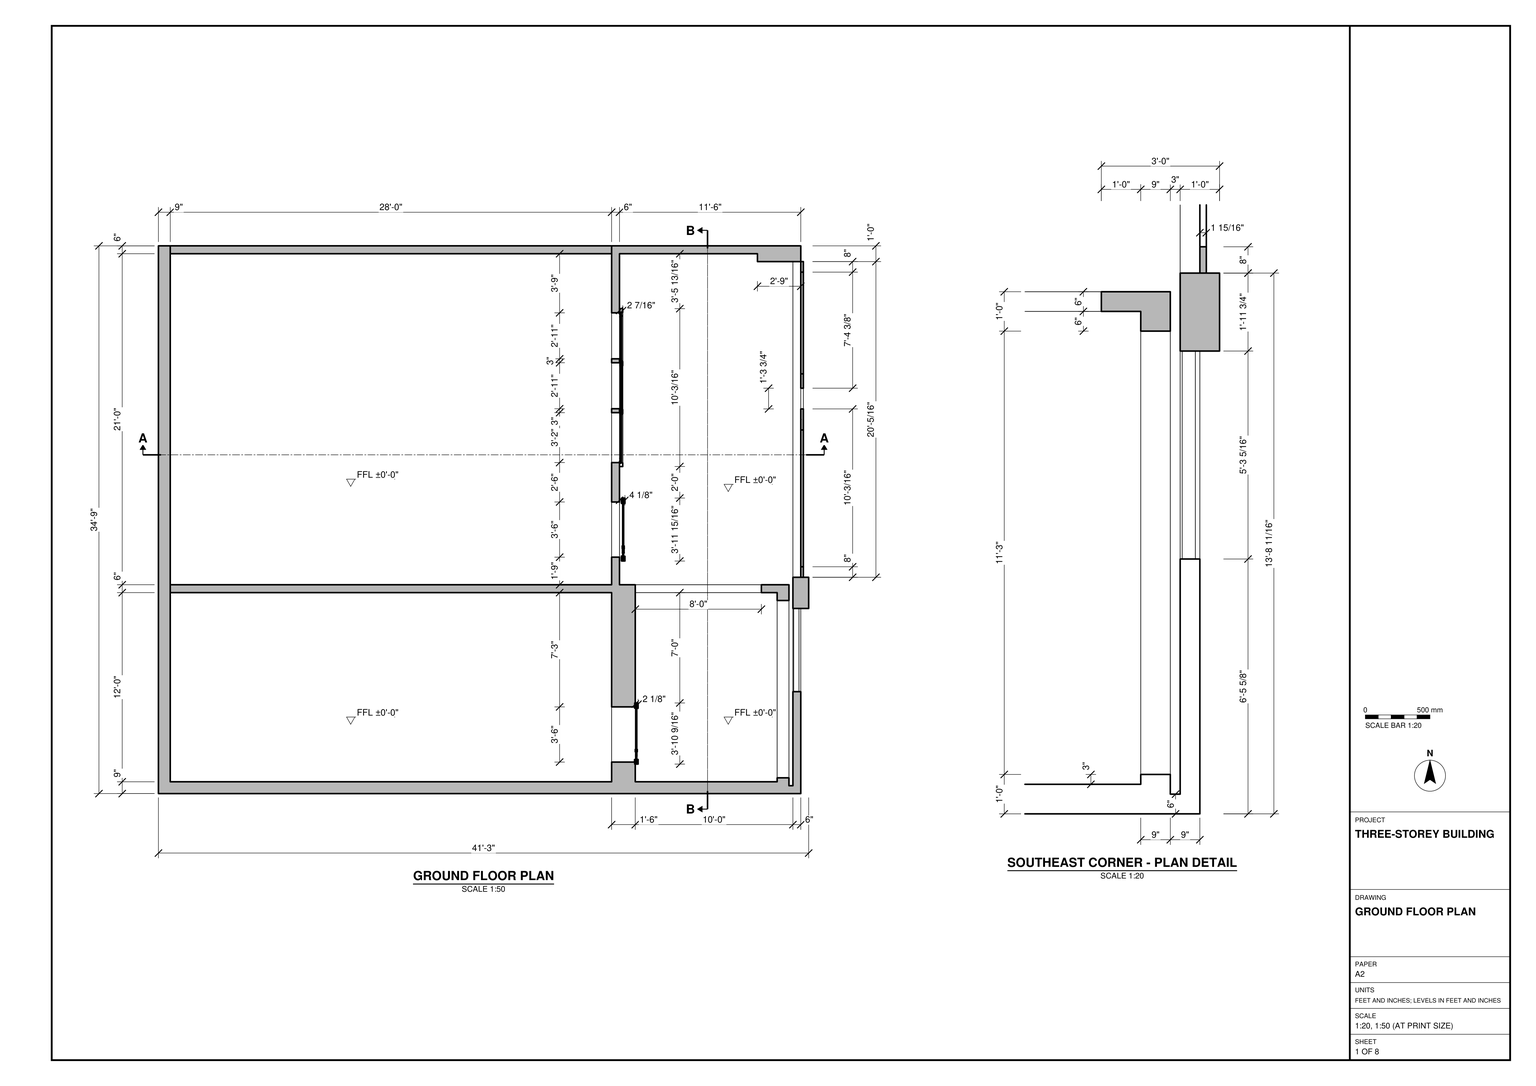
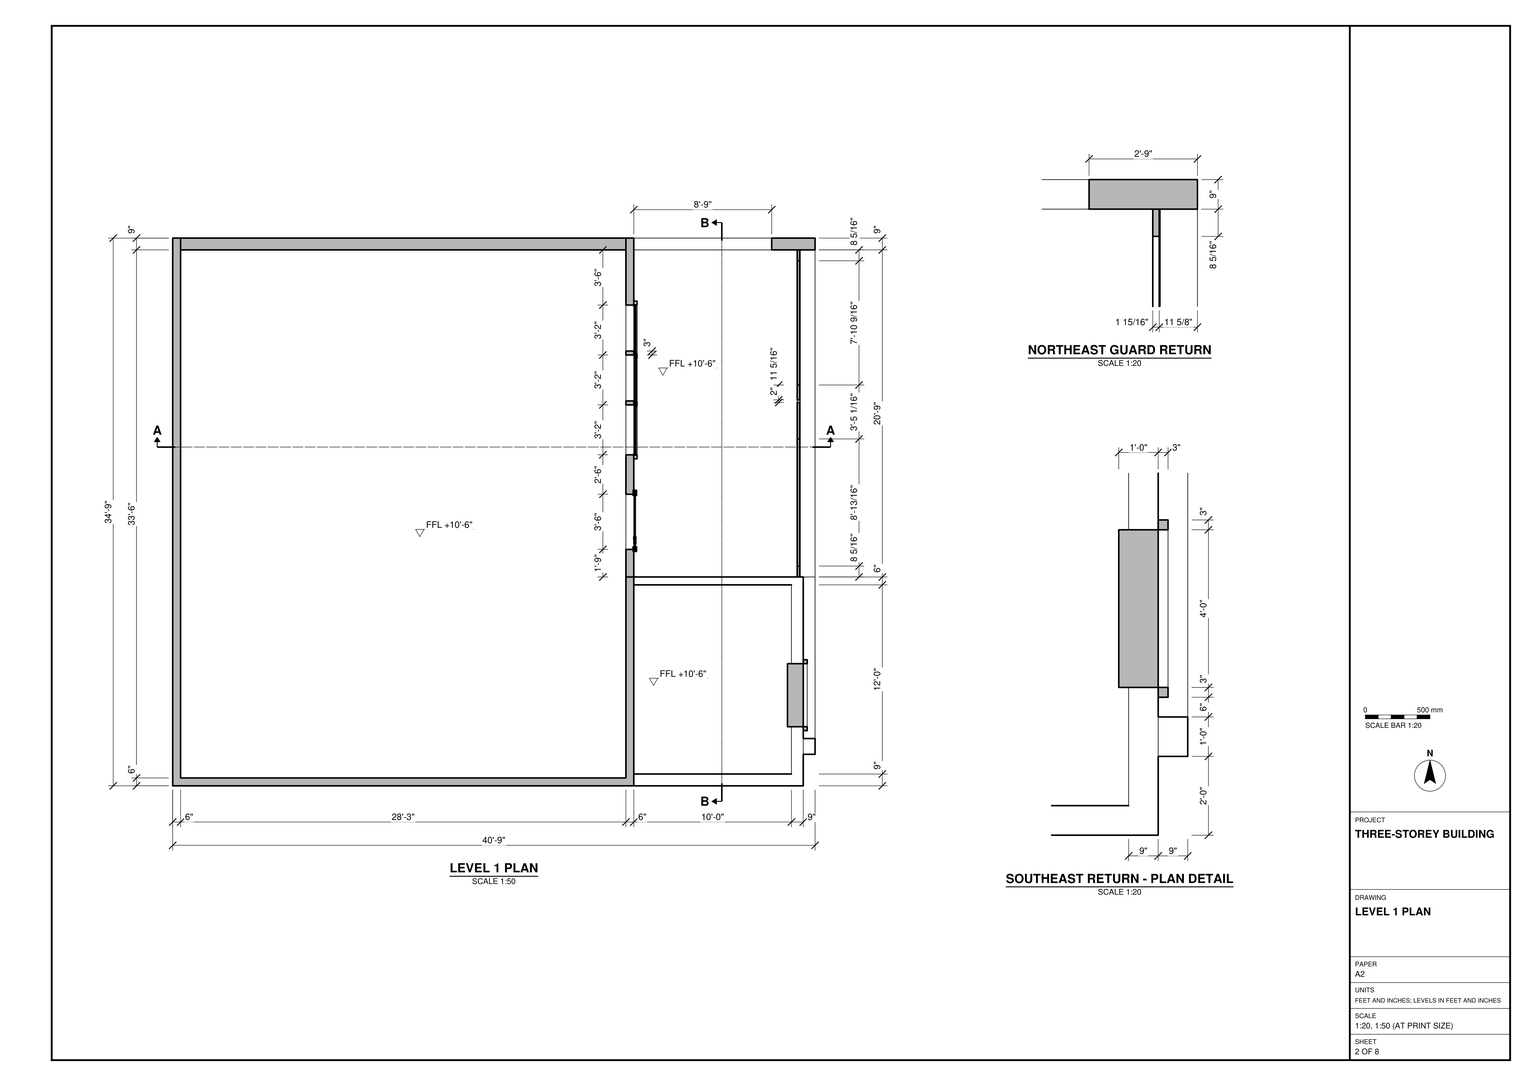
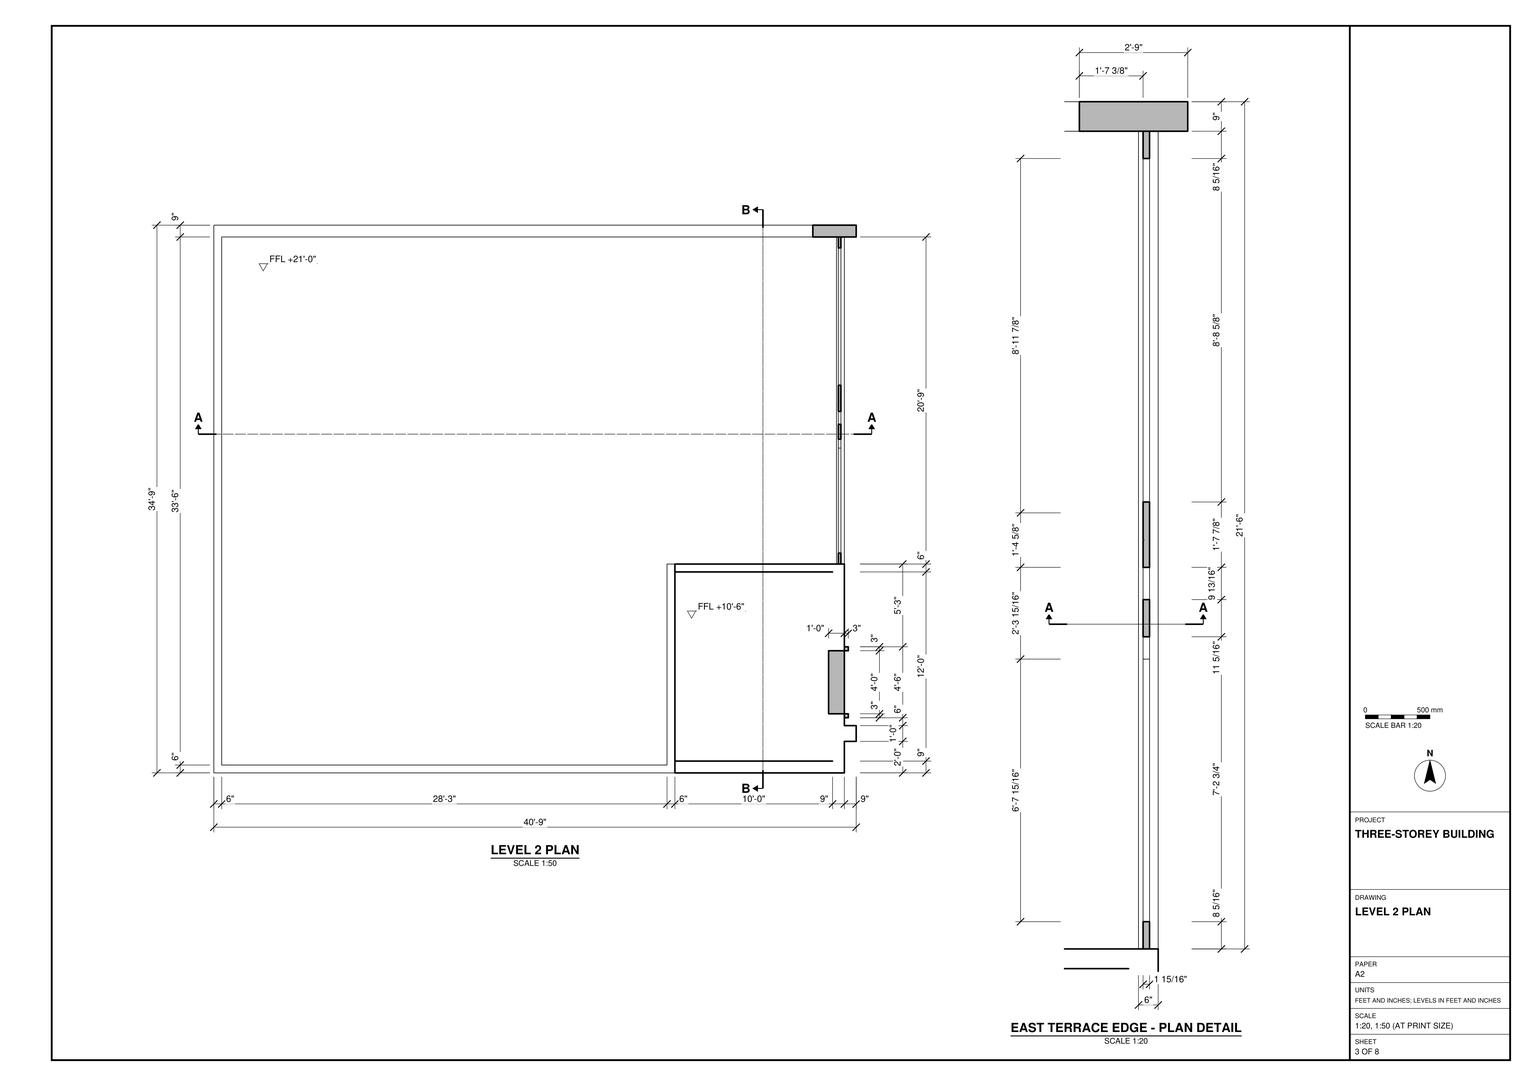
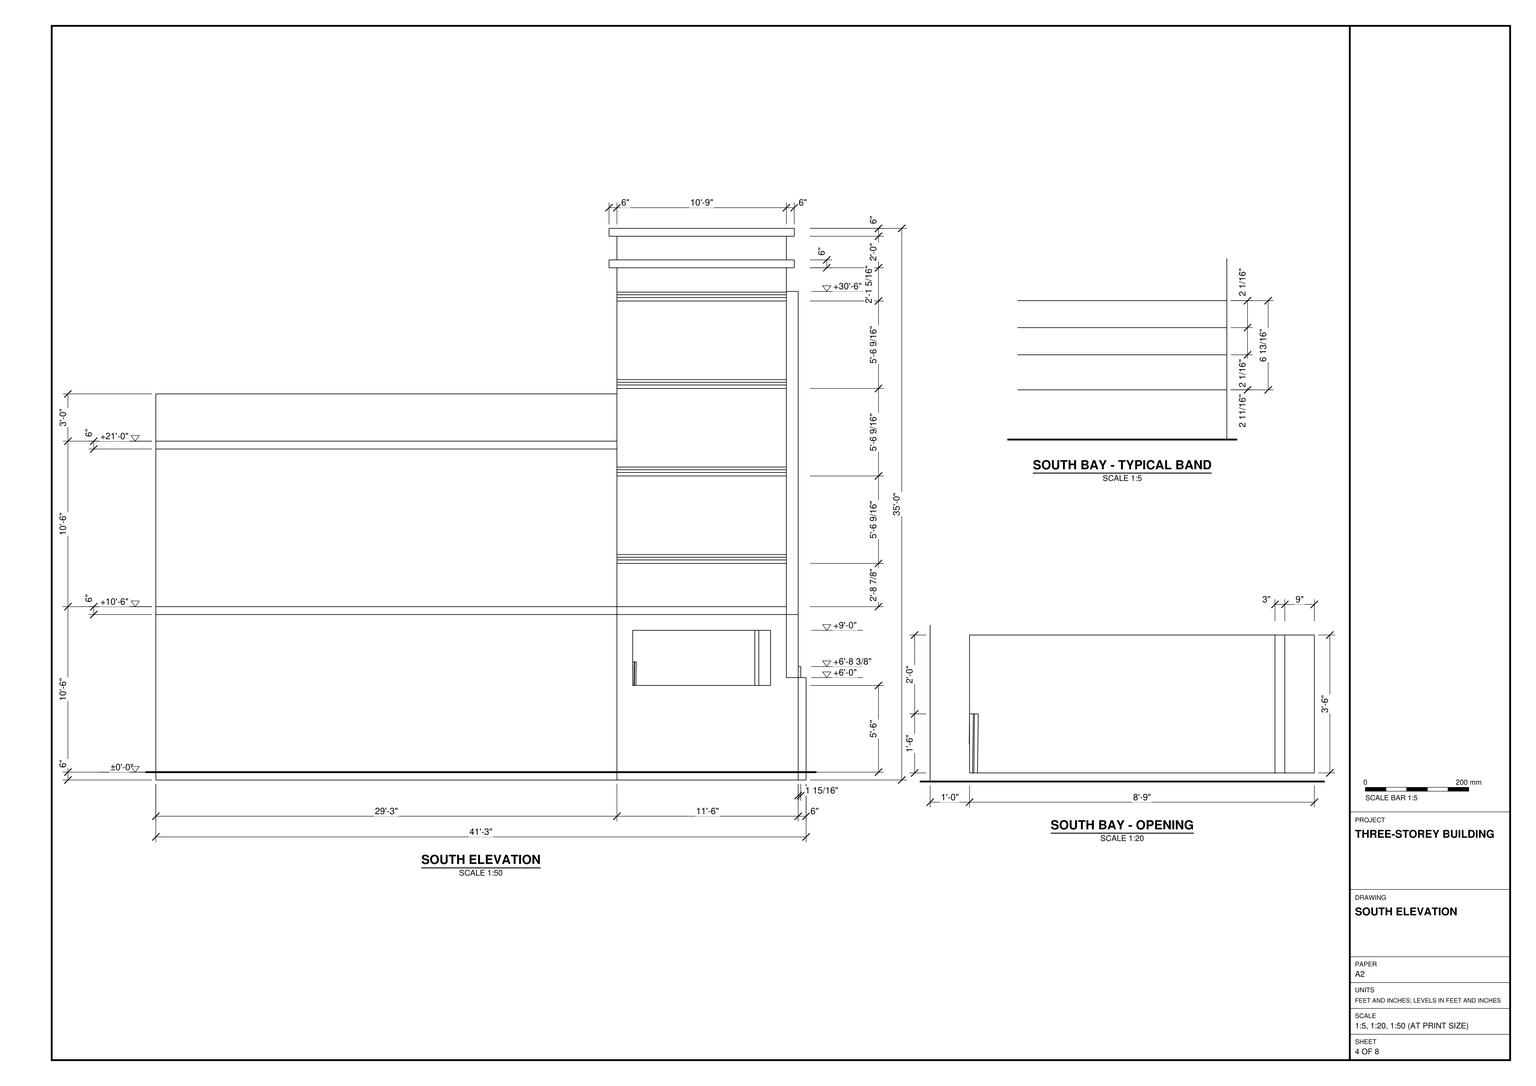
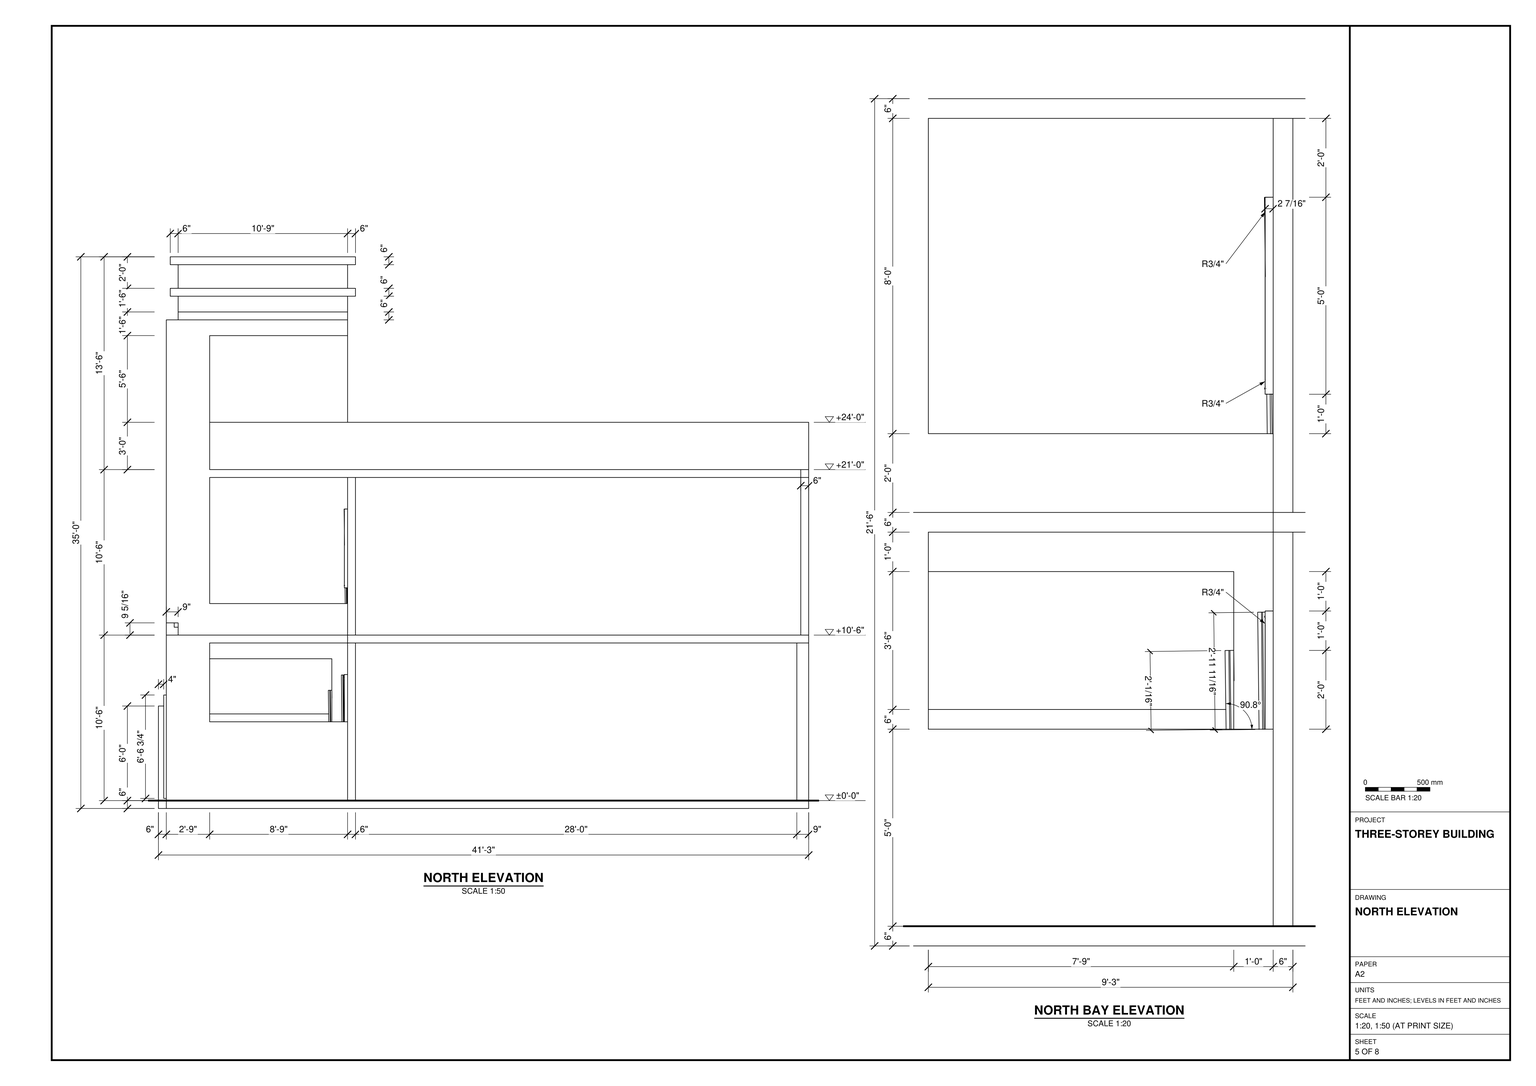
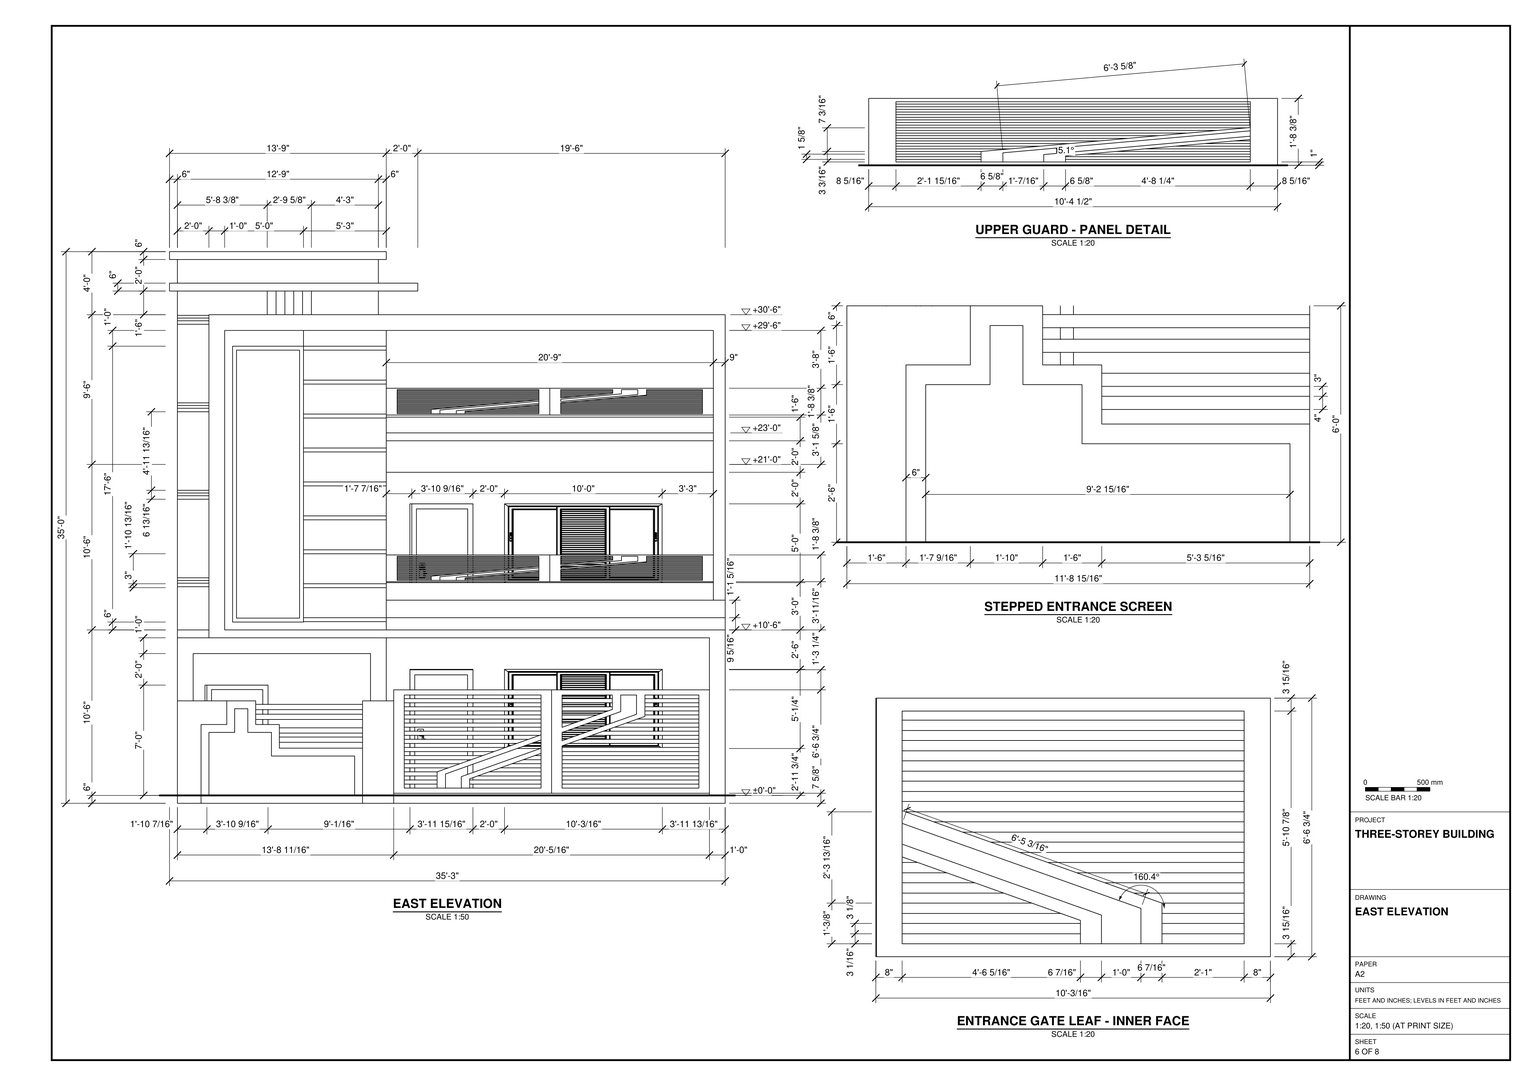
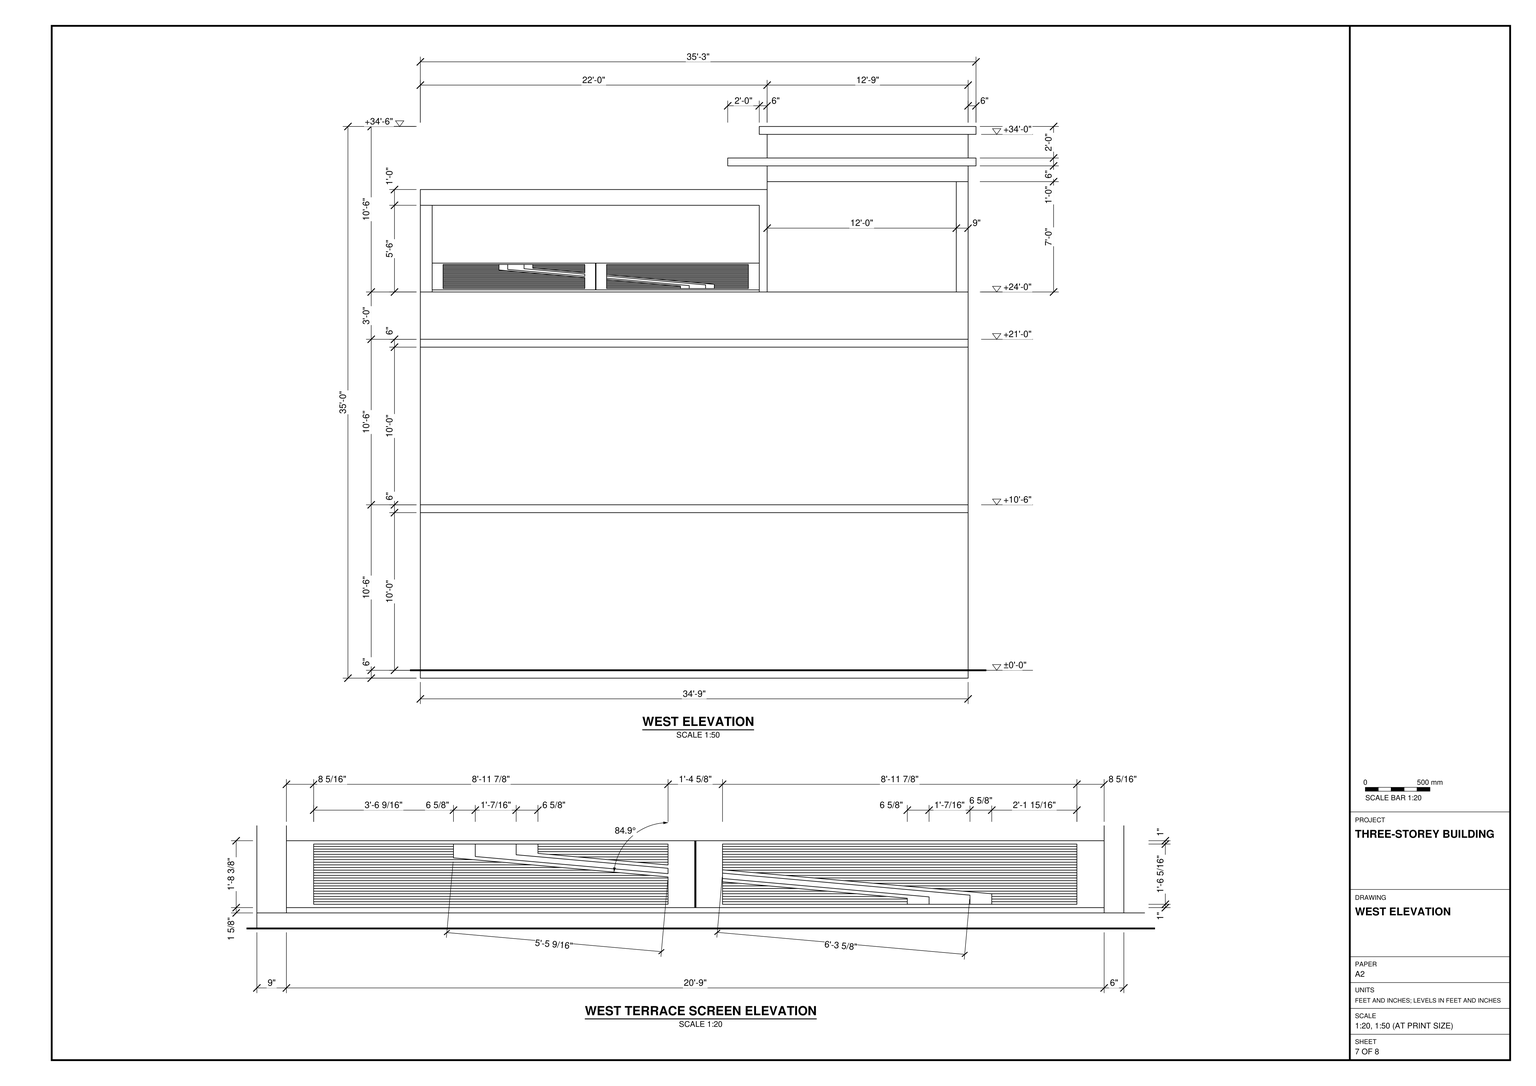
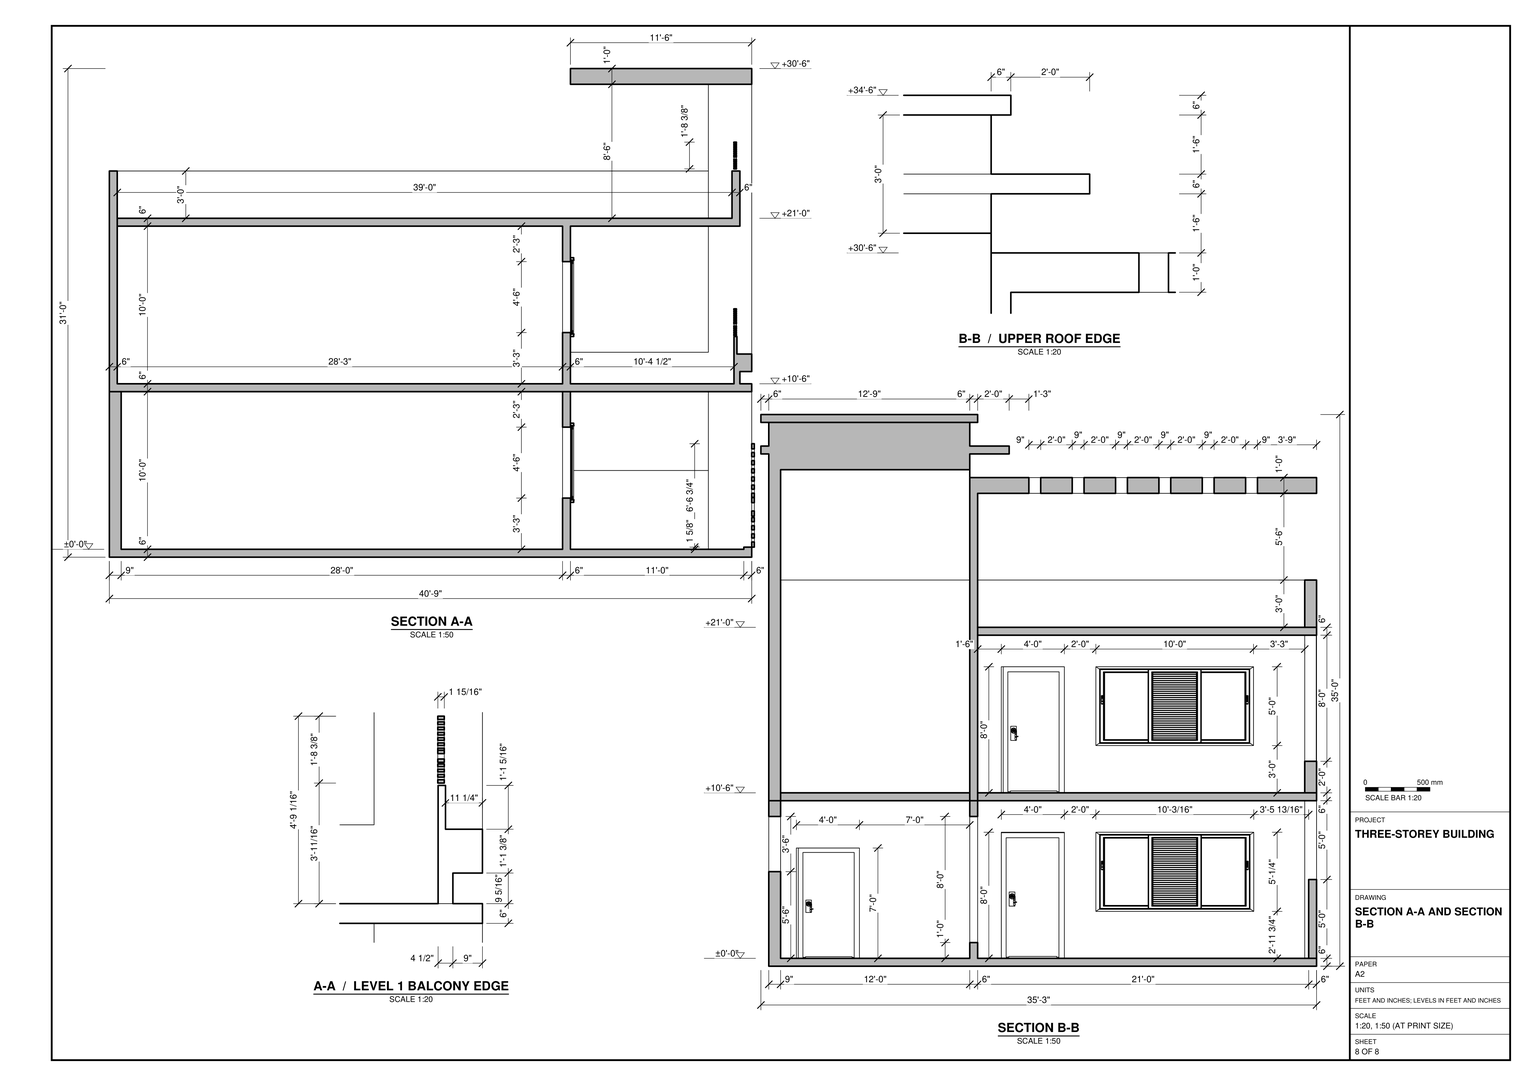
Build the three-storey building in SketchUp from task_files/diagram_01.pdf. Work in feet and inches. The overall extents are 41'-3" east to west, 35'-3" north to south and 35'-0" high. Set the finished floor levels at ±0'-0", +10'-6" and +21'-0".

Lay out the broad western bay and the narrower strip along its east side. On the ground floor, divide the western bay into north and south rooms. On Level 1, leave the western bay undivided. Follow the wall thicknesses on each plan and place the doors and window units in the openings shown. Shape the Level 2 slab around the southeast area so that the lower floor remains visible from above. Use the enlarged details for the ground-floor southeast corner, the guard returns and the terrace edge.

Model the slabs, roof and vertical connections as shown. Include stairs, built-in joinery and main furniture only where indicated. Keep shell elements such as walls, slabs and roof, and each furniture or joinery piece, in separate groups or components. Use components for repeated parts. Decor and loose items may be any suitable library components. Save one SketchUp model as output_files/three_storey_building_with_its_stepped_east_terrace.skp.

# SketchUp Ruby script. Lengths in inches.
U = 1.inch
M = Sketchup.active_model
def pt(a) = Geom::Point3d.new(a.map { |v| v * U })
def face(e, loops, mat)
  f = e.add_face(loops[0].map { |a| pt(a) })
  loops[1..].each { |l| e.add_face(l.map { |a| pt(a) }).erase! }
  f.material = f.back_material = mat if mat
  f
end
# faces: each face lists its corners as indices into pts; further lists are holes
def faces(e, pts, list, mat = nil) = list.each { |f| face(e, (f[0].is_a?(Array) ? f : [f]).map { |l| l.map { |i| pts[i] } }, mat) }
# xy, xz, yz: faces in a plane at the given z, y or x. An outline is a flat list of corners, or four numbers for a rectangle; further outlines are holes
def ring(l) = l.size == 4 ? [[l[0], l[1]], [l[2], l[1]], [l[2], l[3]], [l[0], l[3]]] : l.each_slice(2).to_a
def flat(e, list, mat, &to3) = list.each { |f| face(e, (f[0].is_a?(Array) ? f : [f]).map { |l| ring(l).map { |u, v| to3.(u, v) } }, mat) }
def xy(e, z, list, mat = nil) = flat(e, list, mat) { |x, y| [x, y, z] }
def xz(e, y, list, mat = nil) = flat(e, list, mat) { |x, z| [x, y, z] }
def yz(e, x, list, mat = nil) = flat(e, list, mat) { |y, z| [x, y, z] }
def lines(e, pts, list) = list.each { |a, b| e.add_line(pt(pts[a]), pt(pts[b])) }
# prism: a flat outline (further loops are holes) pulled along v
def prism(e, loops, v, mat = nil)
  f = face(e, loops, mat); d = Geom::Vector3d.new(v.map { |x| x * U })
  f.pushpull(f.normal.samedirection?(d) ? d.length : -d.length)
end
def box(e, o, s, mat = nil) = prism(e, [[o, [o[0] + s[0], o[1], o[2]], [o[0] + s[0], o[1] + s[1], o[2]], [o[0], o[1] + s[1], o[2]]]], [0, 0, s[2]], mat)
def at(x, y, z, deg = 0) = Geom::Transformation.translation(pt([x, y, z])) * Geom::Transformation.rotation(ORIGIN, Z_AXIS, deg.degrees)
def axes(o, x, y, z) = Geom::Transformation.new([*x, 0, *y, 0, *z, 0, *pt(o).to_a, 1])
def part(name) = M.definitions.add(name)
# library, detail: a bought-in or finely detailed component or shape, given as its bounding box
def library(name, o, s) = part(name).tap { |d| box(d.entities, o, s) }
def detail(e, o, s) = box(e.add_group.entities, o, s)
def put(e, d, t, mat = nil) = e.add_instance(d, t).tap { |i| i.material = mat if mat }
def group(e, t, mat = nil) = e.add_group.tap { |g| g.transformation = t; g.material = mat if mat }.entities
root = M.entities
M.materials.add("A08_Garnet_Shadow").color = [102, 0, 0]
M.materials.add("Carpet_04_1K").color = [43, 65, 85]
M.materials.add("D07_Ochre_Flame").color = [153, 107, 0]
M.materials.add("Denim_03_1K").color = [93, 106, 119]
M.materials.add("Glass_Basic_01").color = [14, 101, 186]
M.materials["Glass_Basic_01"].alpha = 0.25
M.materials.add("I01_Sky_Frost").color = [204, 204, 255]
c1 = library("porta+4",[0.2,-5.42,1.33],[46.55,4.72,83.21])
c2 = library("Modern+Gate+1",[0,0,0],[118.11,1.97,78.74])
c3 = library("mesh-160",[-91.39,-1008.79,-36.9],[2366.42,1739.16,65.81])
c4 = part("Group4")
g1 = group(c4.entities,at(-5.75,-6.15,0))
put(g1,c3,axes([0,0,0],[1,0,0],[0,0,1],[0,-1,0]))
p = [[351,423,126],[351,423,0],[351,423,246],[351,414,246]]
lines(root,p,[[0,1],[2,3],[2,0]])
g2 = group(root,at(0,6,0))
xy(g2,-6,[[0,0,0,417,489,417,489,164.68,495,164.68,495,140.93,489,140.93,489,0]])
xy(g2,0,[[480,6,483,6,483,405,456,405,456,411,351,411,351,159,480,159],[9,9,345,153],[363,9,471,153],[9,159,345,411],[456,405,456,411,351,411,351,417,471,417,471,405],
  [471,405,489,417],[9,411,345,417]])
xy(g2,1.64,[[483,164.68,489,405]])
xy(g2,3,[[345,24,363,66],[345,180,351,222]])
xy(g2,6,[[471,12,480,147]])
xy(g2,12,[[363,153,459,159]])
xy(g2,36,[[483,77.61,489,140.93]])
xy(g2,39,[[345,252,351,290],[345,293,351,328],[345,331,351,366]])
xy(g2,40.4375,[[483.62,77.61,487.62,158.93]])
xy(g2,44.4375,[[483.62,77.61,487.62,158.93]])
xy(g2,47.47,[[483.85,77.61,487.85,158.93]])
xy(g2,51.47,[[483.85,77.61,487.85,158.93]])
xy(g2,54,[[483,59.61,489,77.61]])
xy(g2,57.83,[[483.55,59.61,487.55,140.93]])
xy(g2,60,[[351,411,456,417]])
xy(g2,61.83,[[483.55,59.61,487.55,140.93]])
xy(g2,65.33,[[483.55,59.61,487.55,140.93]])
xy(g2,66,[[363,0,468,9]])
xy(g2,69.33,[[483.55,59.61,487.55,140.93]])
xy(g2,72,[[480,0,489,0,489,59.61,483,59.61,483,6,480,6],[483,140.93,489,146.93],[489,140.93,495,140.93,495,164.68,489,164.68,489,158.68,483,158.68,483,146.93,489,146.93],[483,158.68,489,164.68]])
xy(g2,81,[[345,24,363,66]])
xy(g2,93,[[345,180,351,222],[345,252,351,290],[345,293,351,328],[345,331,351,366]])
xy(g2,108,[[363,0,468,9],[471,12,480,147],[363,153,459,159]])
xy(g2,120,[[0,0,351,9],[351,0,480,0,480,159,351,159,351,153,471,153,471,9,351,9],[0,9,9,153],[9,9,345,153],[345,9,351,153],
  [351,9,363,153],[363,9,471,153],[480,24,489,159],[0,153,9,159],[9,153,351,159],
  [0,159,9,417],[9,159,345,411],[345,159,351,417],[351,159,351,417,456,417,456,405,489,405,489,159],[9,411,345,417]])
xy(g2,126,[[6,6,345,408],[351,9,471,153],[480,36,489,159],[351,159,475.5,408],[480,159,489,417],
  [6,408,345,417],[351,408,475.5,417]])
xy(g2,129,[[345,180,351,222]])
xy(g2,132,[[480,42,483,96]])
xy(g2,135,[[480,45,483,93]])
xy(g2,135,[[468,45,480,93]],"I01_Sky_Frost")
xy(g2,135.31,[[480,159,489,417]])
xy(g2,148.66,[[477.75,159,489,408]])
xy(g2,150,[[351,408,456,417]])
xy(g2,162,[[475.5,159,477.75,408]])
xy(g2,165,[[345,252,351,290],[345,293,351,328],[345,331,351,366]])
xy(g2,219,[[345,180,351,222],[345,252,351,290],[345,293,351,328],[345,331,351,366]])
xy(g2,246,[[6,6,345,408],[351,159,351,417,456,417,456,408,480,408,480,159],[345,408,351,417]])
xy(g2,252,[[6,6,345,6,345,159,474,159,474,408,6,408],[6,408,456,417]])
xy(g2,288,[[0,0,351,0,351,159,345,159,345,6,6,6,6,408,456,408,456,417,0,417],[474,159,480,408]])
xy(g2,339,[[480,45,483,93]])
xy(g2,339,[[468,45,480,93]],"I01_Sky_Frost")
xy(g2,342,[[480,42,483,96]])
xy(g2,354,[[480,36,480,159,471,159,471,198,477,198,477,207,471,207,471,231,477,231,477,240,471,240,471,264,477,264,477,273,471,273,471,297,477,297,477,306,471,306,471,330,477,330,477,339,471,339,471,363,477,363,477,372,471,372,471,408,489,408,489,36],[351,159,351,417,456,417,456,408,471,408,471,372,363,372,363,363,471,363,471,339,363,339,363,330,471,330,471,306,363,306,363,297,471,297,471,273,363,273,363,264,471,264,471,240,363,240,363,231,471,231,471,207,363,207,363,198,471,198,471,159],[471,198,477,207],[471,231,477,240],[471,264,477,273],
  [471,297,477,306],[471,330,477,339],[471,363,477,372]])
xy(g2,366,[[480,24,489,153],[351,153,489,186],[[351,186,489,219],[363,198,477,207]],[[351,219,489,252],[363,231,477,240]],[[351,252,489,285],[363,264,477,273]],
  [[351,285,489,318],[363,297,477,306]],[[351,318,489,351],[363,330,477,339]],[[351,351,489,384],[363,363,477,372]],[351,384,489,417]])
xy(g2,372,[[351,9,471,153]])
xy(g2,384,[[345,-6,345,183,471,183,471,153,351,153,351,0,480,0,480,183,486,183,486,-6],[471,153,480,183]])
xy(g2,390,[[[345,-6,486,183],[351,0,480,153]]])
xy(g2,408,[[345,-6,480,0],[480,-6,486,159],[345,0,351,153],[351,0,480,153],[345,153,480,159]])
xy(g2,414,[[345,-6,486,159]])
xz(g2,-6,[[345,384,486,390],[345,408,486,414]])
xz(g2,0,[[0,-6,351,120],[[351,-6,489,-6,489,72,480,72,480,120,351,120],[363,66,468,108]],[0,120,351,126],[351,120,480,126],[0,126,351,246],
  [351,158.9,480,161.57],[351,163.64,480,165.69],[351,225.5,480,228.17],[351,230.23,480,232.29],[0,246,351,252],
  [0,252,351,288],[351,292.09,480,294.76],[351,296.83,480,298.88],[351,358.68,480,361.35],[351,363.42,480,365.47]])
xz(g2,0,[[351,126,480,158.9],[351,161.57,480,163.64],[351,165.69,480,225.5],[351,228.17,480,230.23],[351,232.29,480,292.09],
  [351,294.76,480,296.83],[351,298.88,480,358.68],[351,361.35,480,363.42],[351,365.47,480,384],[351,390,480,408]],"Denim_03_1K")
xz(g2,6,[[480,0,483,72],[6,126,345,246],[6,246,345,252],[6,252,345,288]])
xz(g2,9,[[9,0,345,120],[363,0,363,66,468,66,468,108,363,108,363,120,471,120,471,0],[351,120,471,126],[351,126,471,372]])
xz(g2,12,[[471,6,480,108]])
xz(g2,24,[[345,3,363,81],[480,120,489,366]])
xz(g2,36,[[480,126,489,354]])
xz(g2,42,[[480,132,483,342]])
xz(g2,45,[[480,135,483,339]])
xz(g2,45,[[468,135,480,339]],"I01_Sky_Frost")
xz(g2,59.61,[[[483,54,489,72],[483.55,65.33,487.55,69.33],[483.55,57.83,487.55,61.83]]])
xz(g2,66,[[345,3,363,81]])
xz(g2,77.61,[[[483,36,489,54],[483.85,47.47,487.85,51.47],[483.62,40.4375,487.62,44.4375]]])
xz(g2,93,[[480,135,483,339]])
xz(g2,93,[[468,135,480,339]],"I01_Sky_Frost")
xz(g2,96,[[480,132,483,342]])
xz(g2,140.93,[[[489,-6,495,-6,495,72,483,72,483,36,489,36],[483.55,65.33,487.55,69.33],[483.55,57.83,487.55,61.83]]])
xz(g2,147,[[471,6,480,108]])
xz(g2,153,[[9,0,345,120],[363,0,471,0,471,120,363,120,363,108,459,108,459,12,363,12],[351,120,471,126],[351,126,471,366],[351,366,480,372],
  [351,372,480,384],[351,390,480,408]])
xz(g2,158.93,[[483.62,40.4375,487.62,44.4375],[483.85,47.47,487.85,51.47]])
xz(g2,159,[[9,0,345,120],[[351,0,480,120],[363,12,459,108]],[345,120,351,252],[351,120,471,126],[351,126,351,246,480,246,480,148.66,477.75,148.66,477.75,162,475.5,162,475.5,126],
  [480,135.31,489,148.66],[351,246,471,252],[471,246,480,252],[345,252,351,288],[351,252,351,354,480,354,480,288,474,288,474,252],
  [345,408,486,414]])
xz(g2,164.68,[[489,-6,495,72],[483,1.64,489,72]])
xz(g2,180,[[345,3,351,93],[345,129,351,219]])
xz(g2,183,[[345,384,486,390]])
xz(g2,198,[[363,354,477,366]])
xz(g2,207,[[363,354,477,366]])
xz(g2,222,[[345,3,351,93],[345,129,351,219]])
xz(g2,231,[[363,354,477,366]])
xz(g2,240,[[363,354,477,366]])
xz(g2,252,[[345,39,351,93],[345,165,351,219]])
xz(g2,264,[[363,354,477,366]])
xz(g2,273,[[363,354,477,366]])
xz(g2,290,[[345,39,351,93],[345,165,351,219]])
xz(g2,293,[[345,39,351,93],[345,165,351,219]])
xz(g2,297,[[363,354,477,366]])
xz(g2,306,[[363,354,477,366]])
xz(g2,328,[[345,39,351,93],[345,165,351,219]])
xz(g2,330,[[363,354,477,366]])
xz(g2,331,[[345,39,351,93],[345,165,351,219]])
xz(g2,339,[[363,354,477,366]])
xz(g2,363,[[363,354,477,366]])
xz(g2,366,[[345,39,351,93],[345,165,351,219]])
xz(g2,372,[[363,354,477,366]])
xz(g2,405,[[456,0,483,0,483,1.64,489,1.64,489,120,456,120],[483,0,489,1.64]])
xz(g2,408,[[6,126,345,246],[351,126,475.5,126,475.5,162,477.75,162,477.75,148.66,489,148.66,489,354,456,354,456,252,474,252,474,288,480,288,480,246,456,246,456,150,351,150],[6,252,456,288]])
xz(g2,411,[[9,0,345,120],[351,0,456,60]])
xz(g2,417,[[0,-6,0,120,9,120,9,0,489,0,489,-6],[351,0,351,60,456,60,456,120,0,120,0,126,489,126,489,0],[9,0,345,120],[345,0,351,120],[0,126,6,246],
  [351,126,351,150,456,150,456,246,6,246,6,252,456,252,456,354,351,354,351,366,489,366,489,135.31,480,135.31,480,126],[6,126,345,246],[345,126,351,246],[0,246,6,252],[0,252,456,288]])
yz(g2,0,[[0,-6,417,120],[0,120,417,126],[0,126,417,246],[0,246,417,252],[0,252,417,288]])
yz(g2,6,[[408,126,417,126,417,252,6,252,6,246,408,246],[6,126,408,246],[6,252,408,288]])
yz(g2,9,[[9,0,153,120],[153,0,159,120],[159,0,411,120],[411,0,417,120]])
yz(g2,345,[[[9,0,153,120],[24,3,66,81]],[[159,0,411,120],[180,3,222,93],[252,39,290,93],[293,39,328,93],[331,39,366,93]],[411,0,417,120],[9,120,153,126],[6,126,9,246],
  [9,126,153,246],[153,126,159,246],[[159,126,408,246],[180,129,222,219],[252,165,290,219],[293,165,328,219],[331,165,366,219]],[408,126,417,246],[6,246,9,252],
  [9,246,153,252],[153,246,159,252],[6,252,9,288],[9,252,159,288],[-6,384,183,390],
  [-6,408,159,414]])
yz(g2,351,[[[159,0,177,0,177,96,225,96,225,0,408,0,408,120,159,120],[249,36,369,96]],[[177,0,225,96],[180,3,222,93]],[408,0,411,0,411,60,417,60,417,120,408,120],[[249,36,369,96],[252,39,290,93],[331,39,366,93],[293,39,328,93]],[0,120,9,288],
  [9,120,153,126],[153,120,159,288],[9,126,153,288],[[159,126,177,126,177,222,225,222,225,126,408,126,408,246,159,246],[249,162,369,222]],[[177,126,225,222],[180,129,222,219]],
  [408,126,416.74,150],[416.74,126,417,150],[408,150,416.74,246],[416.74,150,417,246],[[249,162,369,222],[252,165,290,219],[293,165,328,219],[331,165,366,219]],
  [0,288,9,372],[9,288,153,372],[153,288,153,366,417,366,417,354,159,354,159,288],[0,372,153,384],[0,390,153,408]])
yz(g2,363,[[9,0,21,0,21,84,69,84,69,0,153,0,153,120,9,120],[[21,0,69,84],[24,3,66,81]],[153,12,159,108],[0,66,9,108],[198,354,207,366],
  [231,354,240,366],[264,354,273,366],[297,354,306,366],[330,354,339,366],[363,354,372,366]])
yz(g2,456,[[405,0,405,120,417,120,417,60,411,60,411,0],[408,150,417,246],[408,288,417,354]])
yz(g2,459,[[153,12,159,108]])
yz(g2,468,[[0,66,9,108]])
yz(g2,468,[[45,135,93,339]],"I01_Sky_Frost")
yz(g2,471,[[[9,0,153,120],[12,6,147,108]],[9,120,153,126]])
yz(g2,474,[[159,252,408,288]])
yz(g2,475.5,[[159,126,408,162]])
yz(g2,477,[[198,354,207,366],[231,354,240,366],[264,354,273,366],[297,354,306,366],[330,354,339,366],
  [363,354,372,366]])
yz(g2,477.75,[[159,148.66,408,162]])
yz(g2,480,[[[6,0,159,0,159,120,0,120,0,72,6,72],[12,6,147,108]],[0,120,24,126],[96,132.31,159,135.31],[96,158.15,159,161.15],[0,158.9,24,161.57],
  [0,163.64,24,165.69],[96,183.99,159,186.99],[96,209.82,159,212.82],[0,225.5,24,228.17],[0,230.23,24,232.29],
  [96,235.66,159,238.66],[159,246,408,270],[96,261.49,159,264.49],[159,270,408,276],[159,276,408,288],
  [96,287.33,159,290.33],[0,292.09,24,294.76],[0,296.83,24,298.88],[96,313.16,159,316.16],[96,339,159,342],
  [0,358.68,24,361.35],[0,363.42,24,365.47],[68.375,366,75.1,384],[81.83,366,88.56,384],[95.29,366,102.01,384]])
yz(g2,480,[[96,135.31,159,158.15],[96,161.15,159,183.99],[96,186.99,159,209.82],[96,212.82,159,235.66],[96,238.66,159,261.49],
  [96,264.49,159,287.33],[96,290.33,159,313.16],[96,316.16,159,339],[96,342,159,354]],"D07_Ochre_Flame")
yz(g2,480,[[0,126,24,158.9],[36,126,159,126,159,132.31,96,132.31,96,132,42,132,42,342,96,342,96,354,36,354],[159,126,417,135.31],[0,161.57,24,163.64],[0,165.69,24,225.5],
  [0,228.17,24,230.23],[0,232.29,24,292.09],[0,294.76,24,296.83],[0,298.88,24,358.68],[0,361.35,24,363.42],
  [0,365.47,24,365.47,24,366,68.375,366,68.375,384,0,384],[75.1,366,81.83,384],[88.56,366,95.29,384],[102.01,366,153,384],[0,390,153,408]],"Denim_03_1K")
yz(g2,480,[[[42,132,96,342],[45,135,93,339]],[45,135,93,339]],"Glass_Basic_01")
yz(g2,483,[[6,0,6,72,59.61,72,59.61,54,77.61,54,77.61,36,140.93,36,140.93,72,164.68,72,164.68,1.64,405,1.64,405,0],[[42,132,96,342],[45,135,93,339]]])
yz(g2,483.55,[[59.61,57.83,140.93,61.83],[59.61,65.33,140.93,69.33]])
yz(g2,483.62,[[77.61,40.4375,158.93,44.4375]])
yz(g2,483.85,[[77.61,47.47,158.93,51.47]])
yz(g2,486,[[-6,384,183,390],[-6,408,159,414]])
yz(g2,487.55,[[59.61,57.83,140.93,61.83],[59.61,65.33,140.93,69.33]])
yz(g2,487.62,[[77.61,40.4375,158.93,44.4375]])
yz(g2,487.85,[[77.61,47.47,158.93,51.47]])
yz(g2,489,[[0,-6,18,-6,18,54,37.59,54,37.59,72,0,72],[164.68,-6,417,-6,417,0,405,0,405,1.64,164.68,1.64],[405,0,417,0,417,126,36,126,36,354,408,354,408,148.66,417,148.66,417,366,24,366,24,120,405,120],[159,135.31,417,148.66]])
yz(g2,489,[[[18,-6,140.93,-6,140.93,36,77.61,36,77.61,54,59.61,54,59.61,72,37.59,72,37.59,54,18,54],[24,0,24,48,43.59,48,43.59,66,53.61,66,53.61,48,71.61,48,71.61,30,134.93,30,134.93,0]],[24,0,134.93,0,134.93,30,71.61,30,71.61,48,53.61,48,53.61,66,43.59,66,43.59,48,24,48]],"Carpet_04_1K")
yz(g2,495,[[140.93,-6,164.68,72]])
p = [[471,9,372],[480,9,372]]
lines(g2,p,[[0,1]])
put(g2,c1,axes([350.3,176.85,-1.54],[0,1.03,0],[-1,0,0],[0,0,1.15]))
put(g2,c1,axes([348.24,178.25,124.46],[0,1,0],[-1,0,0],[0,0,1.15408]))
put(g2,c1,axes([360.24,22.25,-1.35],[0,1,0],[-1,0,0],[0,0,1.00985]))
put(g2,c2,axes([490.97,164.68,1.64],[0,2.03474,0],[-1,0,0],[0,0,1]),"A08_Garnet_Shadow")
put(g2,c2,axes([477.37,159,289.61],[0,2.1082,0],[-1,0,0],[0,0,0.25877]),"A08_Garnet_Shadow")
put(g2,c2,axes([477.37,159,162.72],[0,2.1082,0],[-1,0,0],[0,0,0.25877]),"A08_Garnet_Shadow")
put(g2,c4,axes([352.21,253.93,196.8],[0,0.05071,0],[-0.03937,0,0],[0,0,0.0345]))
put(g2,c4,axes([352.21,253.93,70.7],[0,0.05079,0],[-0.03937,0,0],[0,0,0.03465]))
